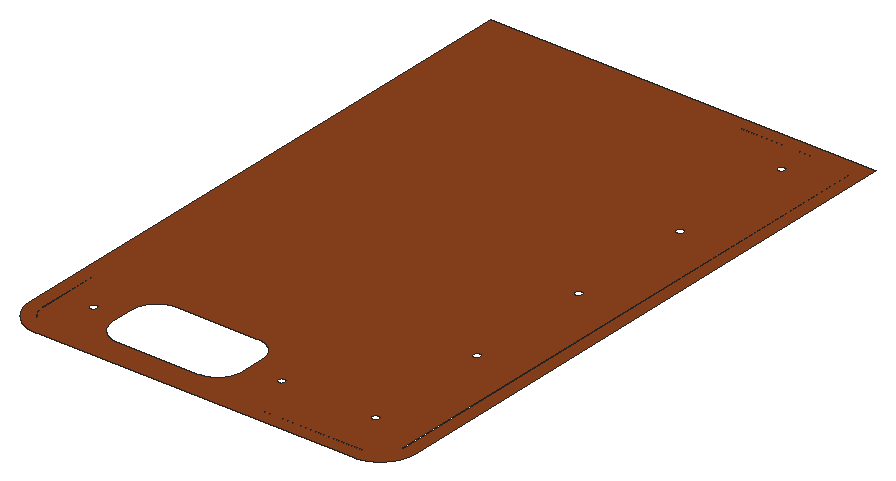
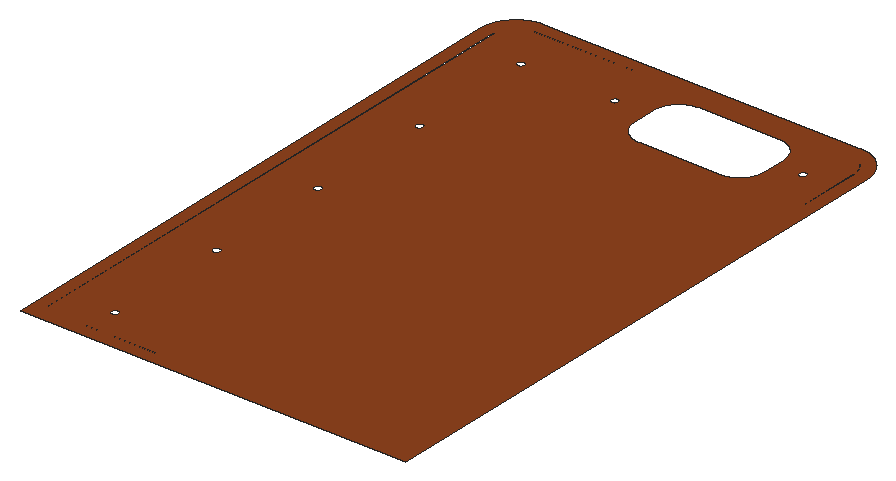
# SketchUp Ruby script. Lengths in inches.
U = 1.inch
M = Sketchup.active_model
def pt(a) = Geom::Point3d.new(a.map { |v| v * U })
def face(e, loops, mat)
  f = e.add_face(loops[0].map { |a| pt(a) })
  loops[1..].each { |l| e.add_face(l.map { |a| pt(a) }).erase! }
  f.material = f.back_material = mat if mat
  f
end
# faces: each face lists its corners as indices into pts; further lists are holes
def faces(e, pts, list, mat = nil) = list.each { |f| face(e, (f[0].is_a?(Array) ? f : [f]).map { |l| l.map { |i| pts[i] } }, mat) }
# xy, xz, yz: faces in a plane at the given z, y or x. An outline is a flat list of corners, or four numbers for a rectangle; further outlines are holes
def ring(l) = l.size == 4 ? [[l[0], l[1]], [l[2], l[1]], [l[2], l[3]], [l[0], l[3]]] : l.each_slice(2).to_a
def flat(e, list, mat, &to3) = list.each { |f| face(e, (f[0].is_a?(Array) ? f : [f]).map { |l| ring(l).map { |u, v| to3.(u, v) } }, mat) }
def xy(e, z, list, mat = nil) = flat(e, list, mat) { |x, y| [x, y, z] }
def xz(e, y, list, mat = nil) = flat(e, list, mat) { |x, z| [x, y, z] }
def yz(e, x, list, mat = nil) = flat(e, list, mat) { |y, z| [x, y, z] }
def lines(e, pts, list) = list.each { |a, b| e.add_line(pt(pts[a]), pt(pts[b])) }
# prism: a flat outline (further loops are holes) pulled along v
def prism(e, loops, v, mat = nil)
  f = face(e, loops, mat); d = Geom::Vector3d.new(v.map { |x| x * U })
  f.pushpull(f.normal.samedirection?(d) ? d.length : -d.length)
end
def box(e, o, s, mat = nil) = prism(e, [[o, [o[0] + s[0], o[1], o[2]], [o[0] + s[0], o[1] + s[1], o[2]], [o[0], o[1] + s[1], o[2]]]], [0, 0, s[2]], mat)
def at(x, y, z, deg = 0) = Geom::Transformation.translation(pt([x, y, z])) * Geom::Transformation.rotation(ORIGIN, Z_AXIS, deg.degrees)
def axes(o, x, y, z) = Geom::Transformation.new([*x, 0, *y, 0, *z, 0, *pt(o).to_a, 1])
def part(name) = M.definitions.add(name)
# library, detail: a bought-in or finely detailed component or shape, given as its bounding box
def library(name, o, s) = part(name).tap { |d| box(d.entities, o, s) }
def detail(e, o, s) = box(e.add_group.entities, o, s)
def put(e, d, t, mat = nil) = e.add_instance(d, t).tap { |i| i.material = mat if mat }
def group(e, t, mat = nil) = e.add_group.tap { |g| g.transformation = t; g.material = mat if mat }.entities
root = M.entities
M.materials.add("[Wood Fence]").color = [142, 67, 30]
xy(root,348,[[[38.66,208,37.98,208.02,36.96,208.08,36.28,208.14,35.94,208.18,35.61,208.22,34.93,208.32,34.6,208.375,34.26,208.44,33.93,208.5,33.59,208.57,33.26,208.64,32.6,208.8,31.94,208.98,31.62,209.07,31.29,209.17,30.97,209.27,30.64,209.38,30.32,209.49,29.68,209.73,29.37,209.85,29.05,209.98,28.74,210.11,28.42,210.25,28.11,210.39,27.81,210.53,27.5,210.68,27.2,210.83,26.89,210.99,26.59,211.15,26.3,211.32,26,211.48,25.71,211.66,25.42,211.83,25.125,212.01,24.84,212.19,24.56,212.38,24.27,212.57,23.99,212.77,23.72,212.97,23.44,213.17,23.17,213.37,22.9,213.58,22.64,213.79,22.11,214.23,21.86,214.45,21.6,214.68,21.1,215.14,20.86,215.375,20.62,215.62,20.375,215.86,20.14,216.1,19.68,216.6,19.45,216.86,19.23,217.11,18.79,217.64,18.58,217.9,18.37,218.17,18.17,218.44,17.97,218.72,17.77,218.99,17.57,219.27,17.38,219.56,17.19,219.84,17.01,220.125,16.83,220.42,16.66,220.71,16.48,221,16.32,221.3,16.15,221.59,15.99,221.89,15.83,222.2,15.68,222.5,15.53,222.81,15.39,223.11,15.25,223.42,15.11,223.74,14.98,224.05,14.85,224.37,14.73,224.68,14.49,225.32,14.38,225.64,14.27,225.97,14.17,226.29,14.07,226.62,13.98,226.94,13.8,227.6,13.64,228.26,13.57,228.59,13.5,228.93,13.44,229.26,13.375,229.6,13.32,229.93,13.22,230.61,13.18,230.94,13.14,231.28,13.08,231.96,13.02,232.98,13,233.66,13,656,296,656,296,233.66,295.98,232.98,295.92,231.96,295.86,231.28,295.82,230.94,295.78,230.61,295.68,229.93,295.625,229.6,295.56,229.26,295.5,228.93,295.43,228.59,295.36,228.26,295.2,227.6,295.02,226.94,294.93,226.62,294.83,226.29,294.73,225.97,294.62,225.64,294.51,225.32,294.27,224.68,294.15,224.37,294.02,224.05,293.89,223.74,293.75,223.42,293.61,223.11,293.47,222.81,293.32,222.5,293.17,222.2,293.01,221.89,292.85,221.59,292.68,221.3,292.52,221,292.34,220.71,292.17,220.42,291.99,220.125,291.81,219.84,291.62,219.56,291.43,219.27,291.23,218.99,291.03,218.72,290.83,218.44,290.63,218.17,290.42,217.9,290.21,217.64,289.77,217.11,289.55,216.86,289.32,216.6,288.86,216.1,288.625,215.86,288.38,215.62,288.14,215.375,287.9,215.14,287.4,214.68,287.14,214.45,286.89,214.23,286.36,213.79,286.1,213.58,285.83,213.37,285.56,213.17,285.28,212.97,285.01,212.77,284.73,212.57,284.44,212.38,284.16,212.19,283.875,212.01,283.58,211.83,283.29,211.66,283,211.48,282.7,211.32,282.41,211.15,282.11,210.99,281.8,210.83,281.5,210.68,281.19,210.53,280.89,210.39,280.58,210.25,280.26,210.11,279.95,209.98,279.63,209.85,279.32,209.73,278.68,209.49,278.36,209.38,278.03,209.27,277.71,209.17,277.38,209.07,277.06,208.98,276.4,208.8,275.74,208.64,275.41,208.57,275.07,208.5,274.74,208.44,274.4,208.375,274.07,208.32,273.39,208.22,273.06,208.18,272.72,208.14,272.04,208.08,271.02,208.02,270.34,208],[82,228,141,228,141.57,228.01,142.13,228.04,142.69,228.08,143.26,228.14,143.82,228.22,144.37,228.32,144.93,228.43,145.48,228.57,146.02,228.71,146.5625,228.88,147.1,229.0625,147.625,229.26,148.15,229.48,148.66,229.71,149.17,229.96,149.67,230.23,150.16,230.51,150.64,230.8,151.12,231.11,151.58,231.4375,152.03,231.78,152.47,232.13,152.9,232.5,153.32,232.88,153.73,233.27,154.12,233.68,154.5,234.1,154.87,234.53,155.22,234.97,155.5625,235.42,155.89,235.88,156.2,236.36,156.49,236.84,156.77,237.33,157.04,237.83,157.29,238.34,157.52,238.85,157.74,239.375,157.9375,239.9,158.12,240.4375,158.29,240.98,158.43,241.52,158.57,242.07,158.68,242.63,158.78,243.18,158.86,243.74,158.92,244.31,158.96,244.87,158.99,245.43,159,246,159,264,158.99,264.57,158.96,265.13,158.92,265.69,158.86,266.26,158.78,266.82,158.68,267.37,158.57,267.93,158.43,268.48,158.29,269.02,158.12,269.5625,157.9375,270.1,157.74,270.625,157.52,271.15,157.29,271.66,157.04,272.17,156.77,272.67,156.49,273.16,156.2,273.64,155.89,274.12,155.5625,274.58,155.22,275.03,154.87,275.47,154.5,275.9,154.12,276.32,153.73,276.73,153.32,277.12,152.9,277.5,152.47,277.87,152.03,278.22,151.58,278.5625,151.12,278.89,150.64,279.2,150.16,279.49,149.67,279.77,149.17,280.04,148.66,280.29,148.15,280.52,147.625,280.74,147.1,280.9375,146.5625,281.12,146.02,281.29,145.48,281.43,144.93,281.57,144.37,281.68,143.82,281.78,143.26,281.86,142.69,281.92,142.13,281.96,141.57,281.99,141,282,82,282,81.43,281.99,80.87,281.96,80.31,281.92,79.74,281.86,79.18,281.78,78.63,281.68,78.07,281.57,77.52,281.43,76.98,281.29,76.4375,281.12,75.9,280.9375,75.375,280.74,74.85,280.52,74.34,280.29,73.83,280.04,73.33,279.77,72.84,279.49,72.36,279.2,71.88,278.89,71.42,278.5625,70.97,278.22,70.53,277.87,70.1,277.5,69.68,277.12,69.27,276.73,68.88,276.32,68.5,275.9,68.13,275.47,67.78,275.03,67.4375,274.58,67.11,274.12,66.8,273.64,66.51,273.16,66.23,272.67,65.96,272.17,65.71,271.66,65.48,271.15,65.26,270.625,65.0625,270.1,64.88,269.5625,64.71,269.02,64.57,268.48,64.43,267.93,64.32,267.37,64.22,266.82,64.14,266.26,64.08,265.69,64.04,265.13,64.01,264.57,64,264,64,246,64.01,245.43,64.04,244.87,64.08,244.31,64.14,243.74,64.22,243.18,64.32,242.63,64.43,242.07,64.57,241.52,64.71,240.98,64.88,240.4375,65.0625,239.9,65.26,239.375,65.48,238.85,65.71,238.34,65.96,237.83,66.23,237.33,66.51,236.84,66.8,236.36,67.11,235.88,67.4375,235.42,67.78,234.97,68.13,234.53,68.5,234.1,68.88,233.68,69.27,233.27,69.68,232.88,70.1,232.5,70.53,232.13,70.97,231.78,71.42,231.4375,71.88,231.11,72.36,230.8,72.84,230.51,73.33,230.23,73.83,229.96,74.34,229.71,74.85,229.48,75.375,229.26,75.9,229.0625,76.4375,228.88,76.98,228.71,77.52,228.57,78.07,228.43,78.63,228.32,79.18,228.22,79.74,228.14,80.31,228.08,80.87,228.04,81.43,228.01],[38.78,217,270.22,217,270.45,217.01,270.67,217.01,270.89,217.02,271.11,217.04,271.33,217.05,271.56,217.07,271.78,217.09,272.22,217.15,272.4375,217.18,272.66,217.21,272.88,217.25,273.1,217.28,273.32,217.33,273.53,217.37,273.97,217.47,274.18,217.52,274.4,217.58,274.61,217.64,274.83,217.7,275.04,217.76,275.46,217.9,275.67,217.98,275.88,218.05,276.51,218.29,276.91,218.47,277.12,218.5625,277.32,218.66,277.52,218.75,277.72,218.85,277.92,218.96,278.11,219.06,278.31,219.17,278.69,219.39,278.88,219.51,279.07,219.62,279.26,219.74,279.44,219.87,279.63,219.99,279.8125,220.12,279.99,220.25,280.35,220.51,280.52,220.65,280.7,220.79,281.04,221.07,281.21,221.22,281.54,221.52,281.86,221.82,282.18,222.14,282.48,222.46,282.78,222.79,282.93,222.96,283.21,223.3,283.35,223.48,283.49,223.65,283.75,224.01,283.88,224.1875,284.01,224.37,284.13,224.56,284.26,224.74,284.38,224.93,284.49,225.12,284.61,225.31,284.83,225.69,284.94,225.89,285.04,226.08,285.15,226.28,285.25,226.48,285.34,226.68,285.4375,226.88,285.53,227.09,285.71,227.49,285.95,228.12,286.02,228.33,286.1,228.54,286.24,228.96,286.3,229.17,286.36,229.39,286.42,229.6,286.48,229.82,286.53,230.03,286.63,230.47,286.67,230.68,286.72,230.9,286.75,231.12,286.79,231.34,286.82,231.5625,286.85,231.78,286.91,232.22,286.93,232.44,286.95,232.67,286.96,232.89,286.98,233.11,286.99,233.33,286.99,233.55,287,233.78,287,647,204,647,204,646,286,646,286,233.79,285.99,233.58,285.99,233.37,285.97,232.95,285.95,232.74,285.93,232.54,285.89,232.12,285.83,231.7,285.8,231.5,285.77,231.29,285.73,231.08,285.69,230.88,285.65,230.67,285.61,230.47,285.56,230.26,285.51,230.0625,285.45,229.86,285.4,229.66,285.22,229.06,285.01,228.46,284.9375,228.27,284.86,228.07,284.78,227.88,284.7,227.68,284.62,227.49,284.35,226.92,284.26,226.74,284.16,226.55,284.0625,226.37,283.96,226.18,283.86,226,283.53,225.46,283.42,225.29,283.3,225.11,283.1875,224.9375,283.07,224.77,282.94,224.6,282.82,224.43,282.69,224.26,282.57,224.09,282.43,223.93,282.17,223.61,281.89,223.29,281.61,222.99,281.46,222.84,281.3125,222.6875,281.16,222.54,281.01,222.39,280.71,222.11,280.39,221.83,280.07,221.57,279.91,221.43,279.74,221.31,279.57,221.18,279.4,221.06,279.23,220.93,279.0625,220.8125,278.89,220.7,278.71,220.58,278.54,220.47,278,220.14,277.82,220.04,277.63,219.9375,277.45,219.84,277.26,219.74,277.08,219.65,276.51,219.38,276.32,219.3,276.12,219.22,275.93,219.14,275.73,219.0625,275.54,218.99,274.94,218.78,274.34,218.6,274.14,218.55,273.9375,218.49,273.74,218.44,273.53,218.39,273.33,218.35,273.12,218.31,272.92,218.27,272.71,218.23,272.5,218.2,272.3,218.17,271.88,218.11,271.46,218.07,271.26,218.05,271.05,218.03,270.63,218.01,270.42,218.01,270.21,218,38.79,218,38.58,218.01,38.37,218.01,37.95,218.03,37.74,218.05,37.54,218.07,37.12,218.11,36.7,218.17,36.5,218.2,36.29,218.23,36.08,218.27,35.88,218.31,35.67,218.35,35.47,218.39,35.26,218.44,35.0625,218.49,34.86,218.55,34.66,218.6,34.06,218.78,33.46,218.99,33.27,219.0625,33.07,219.14,32.88,219.22,32.68,219.3,32.49,219.38,31.92,219.65,31.74,219.74,31.55,219.84,31.37,219.9375,31.18,220.04,31,220.14,30.46,220.47,30.29,220.58,30.11,220.7,29.9375,220.8125,29.77,220.93,29.6,221.06,29.43,221.18,29.26,221.31,29.09,221.43,28.93,221.57,28.61,221.83,28.29,222.11,27.99,222.39,27.84,222.54,27.6875,222.6875,27.54,222.84,27.39,222.99,27.11,223.29,26.83,223.61,26.57,223.93,26.43,224.09,26.31,224.26,26.18,224.43,26.06,224.6,25.93,224.77,25.8125,224.9375,25.7,225.11,25.58,225.29,25.47,225.46,25.14,226,25.04,226.18,24.9375,226.37,24.84,226.55,24.74,226.74,24.65,226.92,24.38,227.49,24.3,227.68,24.22,227.88,24.14,228.07,24.0625,228.27,23.99,228.46,23.78,229.06,23.6,229.66,23.55,229.86,23.49,230.0625,23.44,230.26,23.39,230.47,23.35,230.67,23.31,230.88,23.27,231.08,23.23,231.29,23.2,231.5,23.17,231.7,23.11,232.12,23.07,232.54,23.05,232.74,23.03,232.95,23.01,233.37,23.01,233.58,23,233.79,23,300,22,300,22,233.78,22.01,233.55,22.01,233.33,22.02,233.11,22.04,232.89,22.05,232.67,22.07,232.44,22.09,232.22,22.15,231.78,22.18,231.5625,22.21,231.34,22.25,231.12,22.28,230.9,22.33,230.68,22.37,230.47,22.47,230.03,22.52,229.82,22.58,229.6,22.64,229.39,22.7,229.17,22.76,228.96,22.9,228.54,22.98,228.33,23.05,228.12,23.29,227.49,23.47,227.09,23.5625,226.88,23.66,226.68,23.75,226.48,23.85,226.28,23.96,226.08,24.06,225.89,24.17,225.69,24.39,225.31,24.51,225.12,24.62,224.93,24.74,224.74,24.87,224.56,24.99,224.37,25.12,224.1875,25.25,224.01,25.51,223.65,25.65,223.48,25.79,223.3,26.07,222.96,26.22,222.79,26.52,222.46,26.82,222.14,27.14,221.82,27.46,221.52,27.79,221.22,27.96,221.07,28.3,220.79,28.48,220.65,28.65,220.51,29.01,220.25,29.1875,220.12,29.37,219.99,29.56,219.87,29.74,219.74,29.93,219.62,30.12,219.51,30.31,219.39,30.69,219.17,30.89,219.06,31.08,218.96,31.28,218.85,31.48,218.75,31.68,218.66,31.88,218.5625,32.09,218.47,32.49,218.29,33.12,218.05,33.33,217.98,33.54,217.9,33.96,217.76,34.17,217.7,34.39,217.64,34.6,217.58,34.82,217.52,35.03,217.47,35.47,217.37,35.68,217.33,35.9,217.28,36.12,217.25,36.34,217.21,36.5625,217.18,36.78,217.15,37.22,217.09,37.44,217.07,37.67,217.05,37.89,217.04,38.11,217.02,38.33,217.01,38.55,217.01],[251.84,435,252.16,435,252.24,435.01,252.3125,435.02,252.39,435.03,252.55,435.05,252.625,435.07,252.7,435.08,252.78,435.1,252.85,435.125,252.93,435.15,253,435.17,253.07,435.2,253.15,435.23,253.29,435.29,253.36,435.33,253.43,435.36,253.57,435.44,253.63,435.48,253.7,435.53,253.76,435.57,253.83,435.62,254.01,435.77,254.12,435.88,254.18,435.93,254.38,436.17,254.43,436.24,254.47,436.3,254.52,436.37,254.56,436.43,254.64,436.57,254.67,436.64,254.71,436.71,254.8,436.92,254.83,437,254.85,437.07,254.875,437.15,254.9,437.22,254.92,437.3,254.93,437.375,254.95,437.45,254.97,437.61,254.98,437.6875,254.99,437.76,255,437.84,255,438.16,254.99,438.24,254.98,438.3125,254.97,438.39,254.95,438.55,254.93,438.625,254.92,438.7,254.9,438.78,254.875,438.85,254.85,438.93,254.83,439,254.8,439.07,254.77,439.15,254.71,439.29,254.67,439.36,254.64,439.43,254.56,439.57,254.52,439.63,254.47,439.7,254.43,439.76,254.38,439.83,254.23,440.01,254.12,440.12,254.07,440.18,253.83,440.38,253.76,440.43,253.7,440.47,253.63,440.52,253.57,440.56,253.43,440.64,253.36,440.67,253.29,440.71,253.08,440.8,253,440.83,252.93,440.85,252.85,440.875,252.78,440.9,252.7,440.92,252.625,440.93,252.55,440.95,252.39,440.97,252.3125,440.98,252.24,440.99,252.16,441,251.84,441,251.76,440.99,251.6875,440.98,251.61,440.97,251.45,440.95,251.375,440.93,251.3,440.92,251.22,440.9,251.15,440.875,251.07,440.85,251,440.83,250.93,440.8,250.85,440.77,250.71,440.71,250.64,440.67,250.57,440.64,250.43,440.56,250.37,440.52,250.3,440.47,250.24,440.43,250.17,440.38,249.99,440.23,249.88,440.12,249.82,440.07,249.62,439.83,249.57,439.76,249.53,439.7,249.48,439.63,249.44,439.57,249.36,439.43,249.33,439.36,249.29,439.29,249.2,439.08,249.17,439,249.15,438.93,249.125,438.85,249.1,438.78,249.08,438.7,249.07,438.625,249.05,438.55,249.03,438.39,249.02,438.3125,249.01,438.24,249,438.16,249,437.84,249.01,437.76,249.02,437.6875,249.03,437.61,249.05,437.45,249.07,437.375,249.08,437.3,249.1,437.22,249.125,437.15,249.15,437.07,249.17,437,249.2,436.93,249.23,436.85,249.29,436.71,249.33,436.64,249.36,436.57,249.44,436.43,249.48,436.37,249.53,436.3,249.57,436.24,249.62,436.17,249.77,435.99,249.88,435.88,249.93,435.82,250.17,435.62,250.24,435.57,250.3,435.53,250.37,435.48,250.43,435.44,250.57,435.36,250.64,435.33,250.71,435.29,250.92,435.2,251,435.17,251.07,435.15,251.15,435.125,251.22,435.1,251.3,435.08,251.375,435.07,251.45,435.05,251.61,435.03,251.6875,435.02,251.76,435.01],[251.84,528,252.16,528,252.24,528.01,252.3125,528.02,252.39,528.03,252.55,528.05,252.625,528.07,252.7,528.08,252.78,528.1,252.85,528.125,252.93,528.15,253,528.17,253.07,528.2,253.15,528.23,253.29,528.29,253.36,528.33,253.43,528.36,253.57,528.44,253.63,528.48,253.7,528.53,253.76,528.57,253.83,528.62,254.01,528.77,254.12,528.88,254.18,528.93,254.38,529.17,254.43,529.24,254.47,529.3,254.52,529.37,254.56,529.43,254.64,529.57,254.67,529.64,254.71,529.71,254.8,529.92,254.83,530,254.85,530.07,254.875,530.15,254.9,530.22,254.92,530.3,254.93,530.375,254.95,530.45,254.97,530.61,254.98,530.6875,254.99,530.76,255,530.84,255,531.16,254.99,531.24,254.98,531.3125,254.97,531.39,254.95,531.55,254.93,531.625,254.92,531.7,254.9,531.78,254.875,531.85,254.85,531.93,254.83,532,254.8,532.07,254.77,532.15,254.71,532.29,254.67,532.36,254.64,532.43,254.56,532.57,254.52,532.63,254.47,532.7,254.43,532.76,254.38,532.83,254.23,533.01,254.12,533.12,254.07,533.18,253.83,533.38,253.76,533.43,253.7,533.47,253.63,533.52,253.57,533.56,253.43,533.64,253.36,533.67,253.29,533.71,253.08,533.8,253,533.83,252.93,533.85,252.85,533.875,252.78,533.9,252.7,533.92,252.625,533.93,252.55,533.95,252.39,533.97,252.3125,533.98,252.24,533.99,252.16,534,251.84,534,251.76,533.99,251.6875,533.98,251.61,533.97,251.45,533.95,251.375,533.93,251.3,533.92,251.22,533.9,251.15,533.875,251.07,533.85,251,533.83,250.93,533.8,250.85,533.77,250.71,533.71,250.64,533.67,250.57,533.64,250.43,533.56,250.37,533.52,250.3,533.47,250.24,533.43,250.17,533.38,249.99,533.23,249.88,533.12,249.82,533.07,249.62,532.83,249.57,532.76,249.53,532.7,249.48,532.63,249.44,532.57,249.36,532.43,249.33,532.36,249.29,532.29,249.2,532.08,249.17,532,249.15,531.93,249.125,531.85,249.1,531.78,249.08,531.7,249.07,531.625,249.05,531.55,249.03,531.39,249.02,531.3125,249.01,531.24,249,531.16,249,530.84,249.01,530.76,249.02,530.6875,249.03,530.61,249.05,530.45,249.07,530.375,249.08,530.3,249.1,530.22,249.125,530.15,249.15,530.07,249.17,530,249.2,529.93,249.23,529.85,249.29,529.71,249.33,529.64,249.36,529.57,249.44,529.43,249.48,529.37,249.53,529.3,249.57,529.24,249.62,529.17,249.77,528.99,249.88,528.88,249.93,528.82,250.17,528.62,250.24,528.57,250.3,528.53,250.37,528.48,250.43,528.44,250.57,528.36,250.64,528.33,250.71,528.29,250.92,528.2,251,528.17,251.07,528.15,251.15,528.125,251.22,528.1,251.3,528.08,251.375,528.07,251.45,528.05,251.61,528.03,251.6875,528.02,251.76,528.01],[182.84,249,183.16,249,183.24,249.01,183.3125,249.02,183.39,249.03,183.55,249.05,183.625,249.07,183.7,249.08,183.78,249.1,183.85,249.125,183.93,249.15,184,249.17,184.07,249.2,184.15,249.23,184.29,249.29,184.36,249.33,184.43,249.36,184.57,249.44,184.63,249.48,184.7,249.53,184.76,249.57,184.83,249.62,185.01,249.77,185.12,249.88,185.18,249.93,185.38,250.17,185.43,250.24,185.47,250.3,185.52,250.37,185.56,250.43,185.64,250.57,185.67,250.64,185.71,250.71,185.8,250.92,185.83,251,185.85,251.07,185.875,251.15,185.9,251.22,185.92,251.3,185.93,251.375,185.95,251.45,185.97,251.61,185.98,251.6875,185.99,251.76,186,251.84,186,252.16,185.99,252.24,185.98,252.3125,185.97,252.39,185.95,252.55,185.93,252.625,185.92,252.7,185.9,252.78,185.875,252.85,185.85,252.93,185.83,253,185.8,253.07,185.77,253.15,185.71,253.29,185.67,253.36,185.64,253.43,185.56,253.57,185.52,253.63,185.47,253.7,185.43,253.76,185.38,253.83,185.23,254.01,185.12,254.12,185.07,254.18,184.83,254.38,184.76,254.43,184.7,254.47,184.63,254.52,184.57,254.56,184.43,254.64,184.36,254.67,184.29,254.71,184.08,254.8,184,254.83,183.93,254.85,183.85,254.875,183.78,254.9,183.7,254.92,183.625,254.93,183.55,254.95,183.39,254.97,183.3125,254.98,183.24,254.99,183.16,255,182.84,255,182.76,254.99,182.6875,254.98,182.61,254.97,182.45,254.95,182.375,254.93,182.3,254.92,182.22,254.9,182.15,254.875,182.07,254.85,182,254.83,181.93,254.8,181.85,254.77,181.71,254.71,181.64,254.67,181.57,254.64,181.43,254.56,181.37,254.52,181.3,254.47,181.24,254.43,181.17,254.38,180.99,254.23,180.88,254.12,180.82,254.07,180.62,253.83,180.57,253.76,180.53,253.7,180.48,253.63,180.44,253.57,180.36,253.43,180.33,253.36,180.29,253.29,180.2,253.08,180.17,253,180.15,252.93,180.125,252.85,180.1,252.78,180.08,252.7,180.07,252.625,180.05,252.55,180.03,252.39,180.02,252.3125,180.01,252.24,180,252.16,180,251.84,180.01,251.76,180.02,251.6875,180.03,251.61,180.05,251.45,180.07,251.375,180.08,251.3,180.1,251.22,180.125,251.15,180.15,251.07,180.17,251,180.2,250.93,180.23,250.85,180.29,250.71,180.33,250.64,180.36,250.57,180.44,250.43,180.48,250.37,180.53,250.3,180.57,250.24,180.62,250.17,180.77,249.99,180.88,249.88,180.93,249.82,181.17,249.62,181.24,249.57,181.3,249.53,181.37,249.48,181.43,249.44,181.57,249.36,181.64,249.33,181.71,249.29,181.92,249.2,182,249.17,182.07,249.15,182.15,249.125,182.22,249.1,182.3,249.08,182.375,249.07,182.45,249.05,182.61,249.03,182.6875,249.02,182.76,249.01],[251.84,621,252.16,621,252.24,621.01,252.3125,621.02,252.39,621.03,252.55,621.05,252.625,621.07,252.7,621.08,252.78,621.1,252.85,621.125,252.93,621.15,253,621.17,253.07,621.2,253.15,621.23,253.29,621.29,253.36,621.33,253.43,621.36,253.57,621.44,253.63,621.48,253.7,621.53,253.76,621.57,253.83,621.62,254.01,621.77,254.12,621.88,254.18,621.93,254.38,622.17,254.43,622.24,254.47,622.3,254.52,622.37,254.56,622.43,254.64,622.57,254.67,622.64,254.71,622.71,254.8,622.92,254.83,623,254.85,623.07,254.875,623.15,254.9,623.22,254.92,623.3,254.93,623.375,254.95,623.45,254.97,623.61,254.98,623.6875,254.99,623.76,255,623.84,255,624.16,254.99,624.24,254.98,624.3125,254.97,624.39,254.95,624.55,254.93,624.625,254.92,624.7,254.9,624.78,254.875,624.85,254.85,624.93,254.83,625,254.8,625.07,254.77,625.15,254.71,625.29,254.67,625.36,254.64,625.43,254.56,625.57,254.52,625.63,254.47,625.7,254.43,625.76,254.38,625.83,254.23,626.01,254.12,626.12,254.07,626.18,253.83,626.38,253.76,626.43,253.7,626.47,253.63,626.52,253.57,626.56,253.43,626.64,253.36,626.67,253.29,626.71,253.08,626.8,253,626.83,252.93,626.85,252.85,626.875,252.78,626.9,252.7,626.92,252.625,626.93,252.55,626.95,252.39,626.97,252.3125,626.98,252.24,626.99,252.16,627,251.84,627,251.76,626.99,251.6875,626.98,251.61,626.97,251.45,626.95,251.375,626.93,251.3,626.92,251.22,626.9,251.15,626.875,251.07,626.85,251,626.83,250.93,626.8,250.85,626.77,250.71,626.71,250.64,626.67,250.57,626.64,250.43,626.56,250.37,626.52,250.3,626.47,250.24,626.43,250.17,626.38,249.99,626.23,249.88,626.12,249.82,626.07,249.62,625.83,249.57,625.76,249.53,625.7,249.48,625.63,249.44,625.57,249.36,625.43,249.33,625.36,249.29,625.29,249.2,625.08,249.17,625,249.15,624.93,249.125,624.85,249.1,624.78,249.08,624.7,249.07,624.625,249.05,624.55,249.03,624.39,249.02,624.3125,249.01,624.24,249,624.16,249,623.84,249.01,623.76,249.02,623.6875,249.03,623.61,249.05,623.45,249.07,623.375,249.08,623.3,249.1,623.22,249.125,623.15,249.15,623.07,249.17,623,249.2,622.93,249.23,622.85,249.29,622.71,249.33,622.64,249.36,622.57,249.44,622.43,249.48,622.37,249.53,622.3,249.57,622.24,249.62,622.17,249.77,621.99,249.88,621.88,249.93,621.82,250.17,621.62,250.24,621.57,250.3,621.53,250.37,621.48,250.43,621.44,250.57,621.36,250.64,621.33,250.71,621.29,250.92,621.2,251,621.17,251.07,621.15,251.15,621.125,251.22,621.1,251.3,621.08,251.375,621.07,251.45,621.05,251.61,621.03,251.6875,621.02,251.76,621.01],[44.84,249,45.16,249,45.24,249.01,45.3125,249.02,45.39,249.03,45.55,249.05,45.625,249.07,45.7,249.08,45.78,249.1,45.85,249.125,45.93,249.15,46,249.17,46.07,249.2,46.15,249.23,46.29,249.29,46.36,249.33,46.43,249.36,46.57,249.44,46.63,249.48,46.7,249.53,46.76,249.57,46.83,249.62,47.01,249.77,47.12,249.88,47.18,249.93,47.38,250.17,47.43,250.24,47.47,250.3,47.52,250.37,47.56,250.43,47.64,250.57,47.67,250.64,47.71,250.71,47.8,250.92,47.83,251,47.85,251.07,47.875,251.15,47.9,251.22,47.92,251.3,47.93,251.375,47.95,251.45,47.97,251.61,47.98,251.6875,47.99,251.76,48,251.84,48,252.16,47.99,252.24,47.98,252.3125,47.97,252.39,47.95,252.55,47.93,252.625,47.92,252.7,47.9,252.78,47.875,252.85,47.85,252.93,47.83,253,47.8,253.07,47.77,253.15,47.71,253.29,47.67,253.36,47.64,253.43,47.56,253.57,47.52,253.63,47.47,253.7,47.43,253.76,47.38,253.83,47.23,254.01,47.12,254.12,47.07,254.18,46.83,254.38,46.76,254.43,46.7,254.47,46.63,254.52,46.57,254.56,46.43,254.64,46.36,254.67,46.29,254.71,46.08,254.8,46,254.83,45.93,254.85,45.85,254.875,45.78,254.9,45.7,254.92,45.625,254.93,45.55,254.95,45.39,254.97,45.3125,254.98,45.24,254.99,45.16,255,44.84,255,44.76,254.99,44.6875,254.98,44.61,254.97,44.45,254.95,44.375,254.93,44.3,254.92,44.22,254.9,44.15,254.875,44.07,254.85,44,254.83,43.93,254.8,43.85,254.77,43.71,254.71,43.64,254.67,43.57,254.64,43.43,254.56,43.37,254.52,43.3,254.47,43.24,254.43,43.17,254.38,42.99,254.23,42.88,254.12,42.82,254.07,42.62,253.83,42.57,253.76,42.53,253.7,42.48,253.63,42.44,253.57,42.36,253.43,42.33,253.36,42.29,253.29,42.2,253.08,42.17,253,42.15,252.93,42.125,252.85,42.1,252.78,42.08,252.7,42.07,252.625,42.05,252.55,42.03,252.39,42.02,252.3125,42.01,252.24,42,252.16,42,251.84,42.01,251.76,42.02,251.6875,42.03,251.61,42.05,251.45,42.07,251.375,42.08,251.3,42.1,251.22,42.125,251.15,42.15,251.07,42.17,251,42.2,250.93,42.23,250.85,42.29,250.71,42.33,250.64,42.36,250.57,42.44,250.43,42.48,250.37,42.53,250.3,42.57,250.24,42.62,250.17,42.77,249.99,42.88,249.88,42.93,249.82,43.17,249.62,43.24,249.57,43.3,249.53,43.37,249.48,43.43,249.44,43.57,249.36,43.64,249.33,43.71,249.29,43.92,249.2,44,249.17,44.07,249.15,44.15,249.125,44.22,249.1,44.3,249.08,44.375,249.07,44.45,249.05,44.61,249.03,44.6875,249.02,44.76,249.01],[251.84,249,252.16,249,252.24,249.01,252.3125,249.02,252.39,249.03,252.55,249.05,252.625,249.07,252.7,249.08,252.78,249.1,252.85,249.125,252.93,249.15,253,249.17,253.07,249.2,253.15,249.23,253.29,249.29,253.36,249.33,253.43,249.36,253.57,249.44,253.63,249.48,253.7,249.53,253.76,249.57,253.83,249.62,254.01,249.77,254.12,249.88,254.18,249.93,254.38,250.17,254.43,250.24,254.47,250.3,254.52,250.37,254.56,250.43,254.64,250.57,254.67,250.64,254.71,250.71,254.8,250.92,254.83,251,254.85,251.07,254.875,251.15,254.9,251.22,254.92,251.3,254.93,251.375,254.95,251.45,254.97,251.61,254.98,251.6875,254.99,251.76,255,251.84,255,252.16,254.99,252.24,254.98,252.3125,254.97,252.39,254.95,252.55,254.93,252.625,254.92,252.7,254.9,252.78,254.875,252.85,254.85,252.93,254.83,253,254.8,253.07,254.77,253.15,254.71,253.29,254.67,253.36,254.64,253.43,254.56,253.57,254.52,253.63,254.47,253.7,254.43,253.76,254.38,253.83,254.23,254.01,254.12,254.12,254.07,254.18,253.83,254.38,253.76,254.43,253.7,254.47,253.63,254.52,253.57,254.56,253.43,254.64,253.36,254.67,253.29,254.71,253.08,254.8,253,254.83,252.93,254.85,252.85,254.875,252.78,254.9,252.7,254.92,252.625,254.93,252.55,254.95,252.39,254.97,252.3125,254.98,252.24,254.99,252.16,255,251.84,255,251.76,254.99,251.6875,254.98,251.61,254.97,251.45,254.95,251.375,254.93,251.3,254.92,251.22,254.9,251.15,254.875,251.07,254.85,251,254.83,250.93,254.8,250.85,254.77,250.71,254.71,250.64,254.67,250.57,254.64,250.43,254.56,250.37,254.52,250.3,254.47,250.24,254.43,250.17,254.38,249.99,254.23,249.88,254.12,249.82,254.07,249.62,253.83,249.57,253.76,249.53,253.7,249.48,253.63,249.44,253.57,249.36,253.43,249.33,253.36,249.29,253.29,249.2,253.08,249.17,253,249.15,252.93,249.125,252.85,249.1,252.78,249.08,252.7,249.07,252.625,249.05,252.55,249.03,252.39,249.02,252.3125,249.01,252.24,249,252.16,249,251.84,249.01,251.76,249.02,251.6875,249.03,251.61,249.05,251.45,249.07,251.375,249.08,251.3,249.1,251.22,249.125,251.15,249.15,251.07,249.17,251,249.2,250.93,249.23,250.85,249.29,250.71,249.33,250.64,249.36,250.57,249.44,250.43,249.48,250.37,249.53,250.3,249.57,250.24,249.62,250.17,249.77,249.99,249.88,249.88,249.93,249.82,250.17,249.62,250.24,249.57,250.3,249.53,250.37,249.48,250.43,249.44,250.57,249.36,250.64,249.33,250.71,249.29,250.92,249.2,251,249.17,251.07,249.15,251.15,249.125,251.22,249.1,251.3,249.08,251.375,249.07,251.45,249.05,251.61,249.03,251.6875,249.02,251.76,249.01],[251.84,342,252.16,342,252.24,342.01,252.3125,342.02,252.39,342.03,252.55,342.05,252.625,342.07,252.7,342.08,252.78,342.1,252.85,342.125,252.93,342.15,253,342.17,253.07,342.2,253.15,342.23,253.29,342.29,253.36,342.33,253.43,342.36,253.57,342.44,253.63,342.48,253.7,342.53,253.76,342.57,253.83,342.62,254.01,342.77,254.12,342.88,254.18,342.93,254.38,343.17,254.43,343.24,254.47,343.3,254.52,343.37,254.56,343.43,254.64,343.57,254.67,343.64,254.71,343.71,254.8,343.92,254.83,344,254.85,344.07,254.875,344.15,254.9,344.22,254.92,344.3,254.93,344.375,254.95,344.45,254.97,344.61,254.98,344.6875,254.99,344.76,255,344.84,255,345.16,254.99,345.24,254.98,345.3125,254.97,345.39,254.95,345.55,254.93,345.625,254.92,345.7,254.9,345.78,254.875,345.85,254.85,345.93,254.83,346,254.8,346.07,254.77,346.15,254.71,346.29,254.67,346.36,254.64,346.43,254.56,346.57,254.52,346.63,254.47,346.7,254.43,346.76,254.38,346.83,254.23,347.01,254.12,347.12,254.07,347.18,253.83,347.38,253.76,347.43,253.7,347.47,253.63,347.52,253.57,347.56,253.43,347.64,253.36,347.67,253.29,347.71,253.08,347.8,253,347.83,252.93,347.85,252.85,347.875,252.78,347.9,252.7,347.92,252.625,347.93,252.55,347.95,252.39,347.97,252.3125,347.98,252.24,347.99,252.16,348,251.84,348,251.76,347.99,251.6875,347.98,251.61,347.97,251.45,347.95,251.375,347.93,251.3,347.92,251.22,347.9,251.15,347.875,251.07,347.85,251,347.83,250.93,347.8,250.85,347.77,250.71,347.71,250.64,347.67,250.57,347.64,250.43,347.56,250.37,347.52,250.3,347.47,250.24,347.43,250.17,347.38,249.99,347.23,249.88,347.12,249.82,347.07,249.62,346.83,249.57,346.76,249.53,346.7,249.48,346.63,249.44,346.57,249.36,346.43,249.33,346.36,249.29,346.29,249.2,346.08,249.17,346,249.15,345.93,249.125,345.85,249.1,345.78,249.08,345.7,249.07,345.625,249.05,345.55,249.03,345.39,249.02,345.3125,249.01,345.24,249,345.16,249,344.84,249.01,344.76,249.02,344.6875,249.03,344.61,249.05,344.45,249.07,344.375,249.08,344.3,249.1,344.22,249.125,344.15,249.15,344.07,249.17,344,249.2,343.93,249.23,343.85,249.29,343.71,249.33,343.64,249.36,343.57,249.44,343.43,249.48,343.37,249.53,343.3,249.57,343.24,249.62,343.17,249.77,342.99,249.88,342.88,249.93,342.82,250.17,342.62,250.24,342.57,250.3,342.53,250.37,342.48,250.43,342.44,250.57,342.36,250.64,342.33,250.71,342.29,250.92,342.2,251,342.17,251.07,342.15,251.15,342.125,251.22,342.1,251.3,342.08,251.375,342.07,251.45,342.05,251.61,342.03,251.6875,342.02,251.76,342.01]]],"[Wood Fence]")
